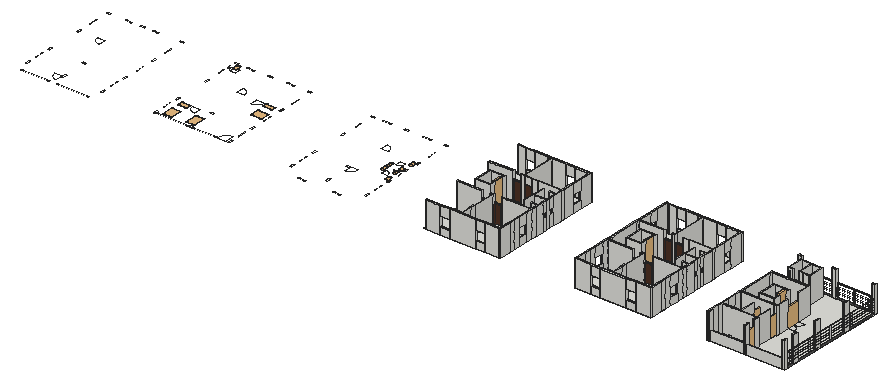
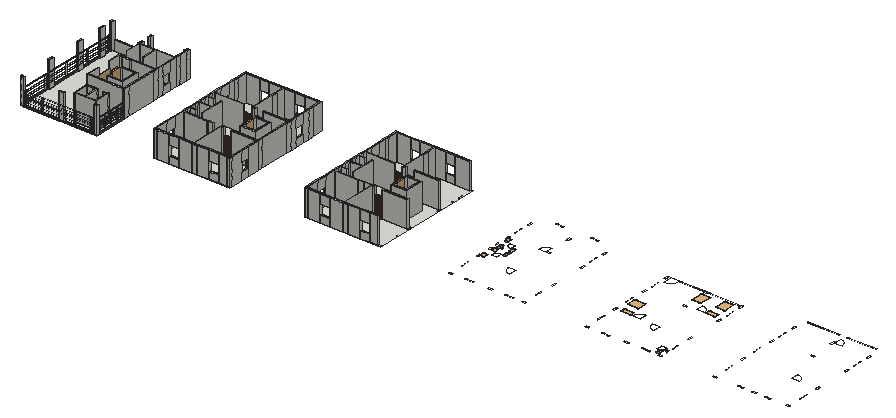
# SketchUp Ruby script. Lengths in inches.
U = 1.inch
M = Sketchup.active_model
def pt(a) = Geom::Point3d.new(a.map { |v| v * U })
def face(e, loops, mat)
  f = e.add_face(loops[0].map { |a| pt(a) })
  loops[1..].each { |l| e.add_face(l.map { |a| pt(a) }).erase! }
  f.material = f.back_material = mat if mat
  f
end
# faces: each face lists its corners as indices into pts; further lists are holes
def faces(e, pts, list, mat = nil) = list.each { |f| face(e, (f[0].is_a?(Array) ? f : [f]).map { |l| l.map { |i| pts[i] } }, mat) }
# xy, xz, yz: faces in a plane at the given z, y or x. An outline is a flat list of corners, or four numbers for a rectangle; further outlines are holes
def ring(l) = l.size == 4 ? [[l[0], l[1]], [l[2], l[1]], [l[2], l[3]], [l[0], l[3]]] : l.each_slice(2).to_a
def flat(e, list, mat, &to3) = list.each { |f| face(e, (f[0].is_a?(Array) ? f : [f]).map { |l| ring(l).map { |u, v| to3.(u, v) } }, mat) }
def xy(e, z, list, mat = nil) = flat(e, list, mat) { |x, y| [x, y, z] }
def xz(e, y, list, mat = nil) = flat(e, list, mat) { |x, z| [x, y, z] }
def yz(e, x, list, mat = nil) = flat(e, list, mat) { |y, z| [x, y, z] }
def lines(e, pts, list) = list.each { |a, b| e.add_line(pt(pts[a]), pt(pts[b])) }
# prism: a flat outline (further loops are holes) pulled along v
def prism(e, loops, v, mat = nil)
  f = face(e, loops, mat); d = Geom::Vector3d.new(v.map { |x| x * U })
  f.pushpull(f.normal.samedirection?(d) ? d.length : -d.length)
end
def box(e, o, s, mat = nil) = prism(e, [[o, [o[0] + s[0], o[1], o[2]], [o[0] + s[0], o[1] + s[1], o[2]], [o[0], o[1] + s[1], o[2]]]], [0, 0, s[2]], mat)
def at(x, y, z, deg = 0) = Geom::Transformation.translation(pt([x, y, z])) * Geom::Transformation.rotation(ORIGIN, Z_AXIS, deg.degrees)
def axes(o, x, y, z) = Geom::Transformation.new([*x, 0, *y, 0, *z, 0, *pt(o).to_a, 1])
def part(name) = M.definitions.add(name)
# library, detail: a bought-in or finely detailed component or shape, given as its bounding box
def library(name, o, s) = part(name).tap { |d| box(d.entities, o, s) }
def detail(e, o, s) = box(e.add_group.entities, o, s)
def put(e, d, t, mat = nil) = e.add_instance(d, t).tap { |i| i.material = mat if mat }
def group(e, t, mat = nil) = e.add_group.tap { |g| g.transformation = t; g.material = mat if mat }.entities
root = M.entities
M.materials.add("JJJ1").color = [238, 218, 183]
M.materials.add("MU TIGHI 6T67L 1").color = [235, 235, 235]
M.materials.add("Polis06_194").color = [79, 50, 36]
M.materials.add("T ER5Y 565N 1").color = [201, 111, 22]
M.materials.add("T R72 56 8, 7 5U1").color = [25, 25, 25]
M.materials.add("wefsd tger 1").color = [92, 92, 92]
c1 = part("bbd")
p = [[-18,-16,0],[-19,-16,0],[18,-16,0],[19,-16,0],[17.2,19.5,0],[14.88,19.37,0],
  [12.57,19.09,0],[10.29,18.67,0],[8.04,18.1,0],[5.83,17.39,0],[3.67,16.53,0],[1.57,15.54,0],
  [-0.46,14.41,0],[-2.41,13.16,0],[-4.28,11.78,0],[-6.0625,10.28,0],[-7.74,8.68,0],[-9.31,6.96,0],
  [-10.76,5.15,0],[-12.1,3.25,0],[-13.31,1.27,0],[-14.39,-0.78,0],[-15.34,-2.9,0],[-16.14,-5.08,0],
  [-16.81,-7.31,0],[-17.33,-9.57,0],[-17.7,-11.86,0],[-17.93,-14.17,0],[-18,-16.5,0],[19.5,-19.5,0],
  [-19.5,-19.5,0],[17,-16.5,0],[18,-16.5,0],[18,19.5,0],[17.2,-16.5,0],[18,-15.5,0],
  [19.5,-15.5,0],[-17,-19.5,0],[-19.5,-15.5,0],[-18,-15.5,0],[-17,-16.5,0],[17,-19.5,0]]
lines(c1.entities,p,[[0,1],[2,3],[4,5],[5,6],[6,7],[7,8],[8,9],[9,10],[10,11],[11,12],[12,13],[13,14],
  [14,15],[15,16],[16,17],[17,18],[18,19],[19,20],[20,21],[21,22],[22,23],[23,24],[24,25],[25,26],
  [26,27],[27,28],[29,30],[31,32],[32,33],[33,4],[4,34],[34,32],[32,35],[35,36],[36,29],[37,30],
  [30,38],[38,39],[39,28],[28,40],[40,37],[31,41],[41,29]])
c2 = part("A$C2CFD65BC")
put(c2.entities,c1,axes([0,0,0],[0.84615,0,0],[0,-0.84615,0],[0,0,0.84615]))
c3 = part("c-1")
p = [[-1.74,-236.76,0],[-12.18,-236.76,0],[-12.18,-260.76,0],[-1.74,-260.76,0],[-184.62,-236.76,0],[-193.62,-236.76,0],
  [-193.62,-260.76,0],[-184.62,-260.76,0],[193.62,-236.76,0],[184.62,-236.76,0],[184.62,-260.76,0],[193.62,-260.76,0],
  [-1.74,-112.8,0],[-1.74,-121.8,0],[-19.74,-121.8,0],[-19.74,-112.8,0],[-175.62,260.76,0],[-175.62,251.76,0],
  [-193.62,251.76,0],[-193.62,260.76,0],[193.62,260.76,0],[193.62,251.76,0],[175.62,251.76,0],[175.62,260.76,0],
  [-1.74,251.76,0],[-1.74,260.76,0],[-25.74,260.76,0],[-25.74,251.76,0],[193.62,-97.8,0],[184.62,-97.8,0],
  [184.62,-121.8,0],[193.62,-121.8,0],[193.62,85.32,0],[184.62,85.32,0],[184.62,61.32,0],[193.62,61.32,0],
  [-184.62,-97.8,0],[-193.62,-97.8,0],[-193.62,-121.8,0],[-184.62,-121.8,0],[-184.62,85.32,0],[-193.62,85.32,0],
  [-193.62,61.32,0],[-184.62,61.32,0]]
lines(c3.entities,p,[[0,1],[1,2],[2,3],[3,0],[4,5],[5,6],[6,7],[7,4],[8,9],[9,10],[10,11],[11,8],
  [12,13],[13,14],[14,15],[15,12],[16,17],[17,18],[18,19],[19,16],[20,21],[21,22],[22,23],[23,20],
  [24,25],[25,26],[26,27],[27,24],[28,29],[29,30],[30,31],[31,28],[32,33],[33,34],[34,35],[35,32],
  [36,37],[37,38],[38,39],[39,36],[40,41],[41,42],[42,43],[43,40]])
c4 = library("A$C064B13D6",[-12.22,-9.4375,0],[24.44,18.875,0.01])
c5 = library("H.F",[-2.42,-4.375,0],[4.84,8.75,0.01])
c6 = library("A$C1C760F31",[-13.95,-18.0625,0],[27.9,36.125,0.01])
c7 = library("A$C4F5E0649",[-23.12,-29.25,0],[46.24,58.5,0.01])
c8 = library("A$C6B07298C",[-24,-12,0],[48,24,0.01])
c9 = library("21''",[-10.5,-8.8125,0],[21,17.625,0.01])
c10 = library("A$C2E2B2BF3",[-14.23,-10.47,0],[28.46,20.94,0.01])
c11 = part("school origo.dwg")
xy(c11.entities,0,[[237.03,315.74,383.625,316.24],[421.44,315.74,584.6,316.24],[1637.66,315.74,1679.3,316.24],[1816.34,315.74,1857.74,316.24],[2364.5625,315.74,2406.2,316.24],
  [2543.24,315.74,2584.64,316.24],[3127,315.74,3168.64,316.24],[3305.68,315.74,3347.08,316.24],[875.22,374.78,1041.66,375.28],[1058.1,374.78,1181.46,375.28],
  [222.16,433.17,222.66,474.57],[600.4,433.17,600.9,474.57],[867.47,433.17,867.97,474.57],[1245.71,433.17,1246.21,474.57],[1556.71,433.17,1557.21,474.57],
  [1934.95,433.17,1935.45,474.57],[2283.61,433.17,2284.11,474.57],[2661.85,433.17,2662.35,474.57],[3046.05,433.17,3046.55,474.57],[3424.29,433.17,3424.79,474.57],
  [3718.02,433.17,3718.52,474.57],[1934.95,581.58,1935.45,599.54],[2661.85,581.58,2662.35,599.54],[3424.29,581.58,3424.79,599.54],[600.4,595.41,600.9,636.81],
  [1245.71,595.41,1246.21,636.81],[1934.95,624.18,1935.45,642.14],[2661.85,624.18,2662.35,642.14],[3424.29,624.18,3424.79,642.14],[222.16,773.125,222.66,814.29],
  [600.4,773.125,600.9,814.29],[1245.71,773.125,1246.21,814.29],[1934.95,773.125,1935.45,814.29],[2661.85,773.125,2662.35,814.29],[3424.29,773.125,3424.79,814.29],
  [867.47,784.33,867.97,814.29],[1556.71,784.33,1557.21,814.29],[2283.61,784.33,2284.11,814.29],[3046.05,784.33,3046.55,814.29],[867.47,835.87,867.97,853.83],
  [315.11,887.3,344.75,887.8],[450.83,887.3,480.23,887.8],[925.02,887.3,966.66,887.8],[1127.1,887.3,1168.5,887.8],[1614.26,887.3,1655.9,887.8],
  [1816.34,887.3,1857.74,887.8],[2341.16,887.3,2382.8,887.8],[2543.24,887.3,2584.64,887.8],[3103.6,887.3,3145.24,887.8],[3305.68,887.3,3347.08,887.8]])
# 6092 loose lines left out
put(c11.entities,c2,axes([3883.4375,490.05,0],[0,1.17818,0],[1.17818,0,0],[0,0,1.17818]))
put(c11.entities,c2,axes([2433.74,727.1,0],[1.18182,0,0],[0,-1.18182,0],[0,0,1.18182]))
put(c11.entities,c2,axes([1763.84,498.99,0],[-1.18182,0,0],[0,1.18182,0],[0,0,1.18182]))
put(c11.entities,c3,at(1746.08,631.29,0))
put(c11.entities,c3,at(3908.89,631.29,0))
put(c11.entities,c3,at(1056.84,631.29,0))
put(c11.entities,c3,at(411.53,631.29,0))
put(c11.entities,c2,axes([333.42,688.11,0],[0,1.18182,0],[1.18182,0,0],[0,0,1.18182]))
put(c11.entities,c2,axes([379.85,360.03,0],[1.18182,0,0],[0,1.18182,0],[0,0,1.18182]))
put(c11.entities,c2,axes([902.52,838.82,0],[0.90909,0,0],[0,-0.90909,0],[0,0,0.90909]))
put(c11.entities,c4,at(894.87,862.82,0,90))
put(c11.entities,c5,axes([875.21,841.2,0],[0,-0.68414,0],[-0.68414,0,0],[0,0,0.68414]))
put(c11.entities,c2,axes([1035.6,727.1,0],[-1.18182,0,0],[0,-1.18182,0],[0,0,1.18182]))
put(c11.entities,c2,axes([1208.46,394.52,0],[1.45455,0,0],[0,-1.45455,0],[0,0,1.45455]))
put(c11.entities,c6,axes([1031.8,427.7,0],[-1.6702,0,0],[0,-1.6702,0],[0,0,1.6702]))
put(c11.entities,c2,axes([972.81,490.07,0],[0,1.17684,0],[1.17684,0,0],[0,0,1.17684]))
put(c11.entities,c7,at(920.83,419.28,0))
put(c11.entities,c8,at(921.75,496.49,0))
put(c11.entities,c2,axes([1763.84,727.1,0],[-1.18182,0,0],[0,-1.18182,0],[0,0,1.18182]))
put(c11.entities,c9,axes([1912.68,631.8,0],[0,1,0],[1,0,0],[0,0,1]))
put(c11.entities,c5,axes([1927.7,624.29,0],[0.68414,0,0],[0,-0.68414,0],[0,0,0.68414]))
put(c11.entities,c10,axes([1921.87,536.4375,0],[0,0.84313,0],[0.84313,0,0],[0,0,0.84313]))
put(c11.entities,c9,axes([1912.72,594.3,0],[0,-1,0],[-1,0,0],[0,0,1]))
put(c11.entities,c5,axes([1897.7,601.8,0],[-0.68414,0,0],[0,0.68414,0],[0,0,0.68414]))
put(c11.entities,c2,axes([1885.7,569.48,0],[-0.90909,0,0],[0,-0.90909,0],[0,0,0.90909]))
put(c11.entities,c2,axes([3920.65,631.05,0],[0,1.09091,0],[-1.09091,0,0],[0,0,1.09091]))
put(c11.entities,c2,axes([3920.65,595.05,0],[0,-1.09091,0],[-1.09091,0,0],[0,0,1.09091]))
put(c11.entities,c2,axes([1137.96,688.11,0],[0,1.18182,0],[-1.18182,0,0],[0,0,1.18182]))
put(c11.entities,c7,at(1201.71,623.01,0,90))
put(c11.entities,c8,axes([1191.82,693.61,0],[-1,0,0],[0,1,0],[0,0,1]))
put(c11.entities,c2,axes([1885.7,656.61,0],[-0.90909,0,0],[0,0.90909,0],[0,0,0.90909]))
put(c11.entities,c10,axes([1921.87,689.56,0],[0,0.84313,0],[0.84313,0,0],[0,0,0.84313]))
put(c11.entities,c10,axes([1854.72,593.92,0],[0,0.84313,0],[0.84313,0,0],[0,0,0.84313]))
put(c11.entities,c10,axes([1854.72,632.17,0],[0,-0.84313,0],[0.84313,0,0],[0,0,0.84313]))
put(c11.entities,c2,axes([2490.74,498.99,0],[-1.18182,0,0],[0,1.18182,0],[0,0,1.18182]))
put(c11.entities,c3,at(2472.98,631.29,0))
put(c11.entities,c2,axes([2490.74,727.1,0],[-1.18182,0,0],[0,-1.18182,0],[0,0,1.18182]))
put(c11.entities,c9,axes([2639.58,631.8,0],[0,1,0],[1,0,0],[0,0,1]))
put(c11.entities,c5,axes([2654.6,624.29,0],[0.68414,0,0],[0,-0.68414,0],[0,0,0.68414]))
put(c11.entities,c10,axes([2648.77,536.4375,0],[0,0.84313,0],[0.84313,0,0],[0,0,0.84313]))
put(c11.entities,c9,axes([2639.625,594.3,0],[0,-1,0],[-1,0,0],[0,0,1]))
put(c11.entities,c5,axes([2624.6,601.8,0],[-0.68414,0,0],[0,0.68414,0],[0,0,0.68414]))
put(c11.entities,c2,axes([2612.6,569.48,0],[-0.90909,0,0],[0,-0.90909,0],[0,0,0.90909]))
put(c11.entities,c2,axes([2612.6,656.61,0],[-0.90909,0,0],[0,0.90909,0],[0,0,0.90909]))
put(c11.entities,c10,axes([2648.77,689.56,0],[0,0.84313,0],[0.84313,0,0],[0,0,0.84313]))
put(c11.entities,c10,axes([2581.62,593.92,0],[0,0.84313,0],[0.84313,0,0],[0,0,0.84313]))
put(c11.entities,c10,axes([2581.62,632.17,0],[0,-0.84313,0],[0.84313,0,0],[0,0,0.84313]))
put(c11.entities,c2,axes([2433.74,498.99,0],[1.18182,0,0],[0,1.18182,0],[0,0,1.18182]))
put(c11.entities,c2,axes([3196.18,727.1,0],[1.18182,0,0],[0,-1.18182,0],[0,0,1.18182]))
put(c11.entities,c2,axes([3253.18,498.99,0],[-1.18182,0,0],[0,1.18182,0],[0,0,1.18182]))
put(c11.entities,c3,at(3235.42,631.29,0))
put(c11.entities,c2,axes([3253.18,727.1,0],[-1.18182,0,0],[0,-1.18182,0],[0,0,1.18182]))
put(c11.entities,c9,axes([3402.01,631.8,0],[0,1,0],[1,0,0],[0,0,1]))
put(c11.entities,c5,axes([3417.04,624.29,0],[0.68414,0,0],[0,-0.68414,0],[0,0,0.68414]))
put(c11.entities,c10,axes([3411.2,536.4375,0],[0,0.84313,0],[0.84313,0,0],[0,0,0.84313]))
put(c11.entities,c9,axes([3402.06,594.3,0],[0,-1,0],[-1,0,0],[0,0,1]))
put(c11.entities,c5,axes([3387.04,601.8,0],[-0.68414,0,0],[0,0.68414,0],[0,0,0.68414]))
put(c11.entities,c2,axes([3375.04,569.48,0],[-0.90909,0,0],[0,-0.90909,0],[0,0,0.90909]))
put(c11.entities,c2,axes([3375.04,656.61,0],[-0.90909,0,0],[0,0.90909,0],[0,0,0.90909]))
put(c11.entities,c10,axes([3411.2,689.56,0],[0,0.84313,0],[0.84313,0,0],[0,0,0.84313]))
put(c11.entities,c10,axes([3344.05,593.92,0],[0,0.84313,0],[0.84313,0,0],[0,0,0.84313]))
put(c11.entities,c10,axes([3344.05,632.17,0],[0,-0.84313,0],[0.84313,0,0],[0,0,0.84313]))
put(c11.entities,c2,axes([3196.18,498.99,0],[1.18182,0,0],[0,1.18182,0],[0,0,1.18182]))
put(c11.entities,c2,axes([3884.88,352.53,0],[0,1.09091,0],[1.09091,0,0],[0,0,1.09091]))
put(c11.entities,c2,axes([3783.02,797.04,0],[0.90909,0,0],[0,-0.90909,0],[0,0,0.90909]))
put(c11.entities,c2,axes([3836.02,797.04,0],[0.90909,0,0],[0,-0.90909,0],[0,0,0.90909]))
put(c11.entities,c4,at(3774.52,837.82,0,90))
put(c11.entities,c5,axes([3754.02,816.2,0],[0,-0.68414,0],[-0.68414,0,0],[0,0,0.68414]))
put(c11.entities,c4,at(3827.52,837.82,0,90))
put(c11.entities,c5,axes([3807.02,816.2,0],[0,-0.68414,0],[-0.68414,0,0],[0,0,0.68414]))
put(c11.entities,c2,axes([3801.14,490.05,0],[0,1.17818,0],[1.17818,0,0],[0,0,1.17818]))
c12 = library("lift",[-933.37,365.14,432],[57.92,12.32,108.27])
c13 = part("Group\#210")
box(c13.entities,[0,0,0],[12,46.92,6])
c14 = part("Flush door assembly \#1")
xy(c14.entities,0,[[0,0,4.72,1.18],[0,34.25,4.72,35.43]],"Polis06_194")
xy(c14.entities,85.26,[[0,1.18,4.72,34.25]],"Polis06_194")
xy(c14.entities,86.61,[[0,0,4.72,35.43]],"Polis06_194")
xz(c14.entities,0,[[0,0,4.72,86.61]],"Polis06_194")
xz(c14.entities,1.18,[[0,0,2.36,85.26],[2.36,0,4.72,85.26]],"Polis06_194")
xz(c14.entities,34.25,[[0,0,4.72,85.26]],"Polis06_194")
xz(c14.entities,35.43,[[0,0,4.72,86.61]],"Polis06_194")
yz(c14.entities,0,[[0,0,1.18,86.61],[34.25,0,35.43,86.61],[1.18,85.26,34.25,86.61]],"Polis06_194")
yz(c14.entities,2.36,[[1.18,0,34.25,0,34.25,85.21,1.18,85.26]],"Polis06_194")
yz(c14.entities,4.72,[[0,0,1.18,86.61],[34.25,0,35.43,86.61],[1.18,85.26,34.25,86.61]],"Polis06_194")
c15 = library("Flush door assembly",[0,0,0],[5.12,30.08,83.9375])
c16 = part("Group\#154")
box(c16.entities,[0,0,0],[12,46.92,6])
c17 = part("Box01")
box(c17.entities,[-251.12,-5.93,-8.91],[582.61,12.27,8.91],"wefsd tger 1")
c18 = part("Box45")
box(c18.entities,[-240.91,-0.82,12.1],[2.44,1.82,74.48],"JJJ1")
c19 = part("Cylinder01")
prism(c19.entities,[[[328.21,-1.16,98.56],[328.21,-0.34,98.26],[328.21,0.53,98.26],[328.21,1.34,98.56],[328.21,2.01,99.11],[328.21,2.44,99.87],[328.21,2.59,100.72],[328.21,2.44,101.58],[328.21,2.01,102.33],[328.21,1.34,102.89],[328.21,0.53,103.18],[328.21,-0.34,103.18],[328.21,-1.16,102.89],[328.21,-1.82,102.33],[328.21,-2.25,101.58],[328.21,-2.41,100.72],[328.21,-2.25,99.87],[328.21,-1.82,99.11]]],[-576.3,0,0],"T ER5Y 565N 1")
c20 = part("Cylinder02")
prism(c20.entities,[[[-239.93,0.18,76.32],[-239.93,0.34,76.26],[-239.93,0.48,76.15],[-239.93,0.5625,75.99],[-239.93,0.59,75.82],[-239.93,0.5625,75.65],[-239.93,0.48,75.5],[-239.93,0.34,75.39],[-239.93,0.18,75.33],[-239.93,0.01,75.33],[-239.93,-0.16,75.39],[-239.93,-0.29,75.5],[-239.93,-0.375,75.65],[-239.93,-0.41,75.82],[-239.93,-0.375,75.99],[-239.93,-0.29,76.15],[-239.93,-0.16,76.26],[-239.93,0.01,76.32]]],[560.05,0,0],"T R72 56 8, 7 5U1")
c21 = part("Rectangle1")
prism(c21.entities,[[[-237.41,1.91,10.08],[-239.22,1.91,10.08],[-239.22,1.91,0.02],[-240.41,1.91,0.02],[-240.41,1.91,10.08],[-242.22,1.91,10.08],[-242.22,1.91,89.41],[-240.41,1.91,89.41],[-240.41,1.91,99.1875],[-239.22,1.91,99.1875],[-239.22,1.91,89.41],[-237.41,1.91,89.41]],[[-240.4375,1.91,85.68],[-240.4375,1.91,13.53],[-239.08,1.91,13.53],[-239.08,1.91,85.68]]],[0,-3.64,0],"MU TIGHI 6T67L 1")
c22 = part("skp243")
put(c22.entities,c17,at(0,0,0))
put(c22.entities,c18,at(0,0,0))
put(c22.entities,c19,at(0,0,0))
put(c22.entities,c20,at(0,0,0))
put(c22.entities,c21,at(0,0,0))
put(c22.entities,c20,at(0,0,-17.07))
put(c22.entities,c20,at(0,0,-35.38))
put(c22.entities,c20,at(0,0,-53.15))
put(c22.entities,c18,at(139.83,0,0))
put(c22.entities,c21,at(139.83,0,0))
put(c22.entities,c21,at(279.78,0,0))
put(c22.entities,c18,at(279.78,0,0))
put(c22.entities,c18,at(419.57,0,0))
put(c22.entities,c21,at(419.57,0,0))
put(c22.entities,c21,at(561.11,0,0))
put(c22.entities,c18,at(561.11,0,0))
c23 = part("Railing1 (1)")
put(c23.entities,c22,at(251.12,5.93,8.91))
c24 = part("Group\#105")
box(c24.entities,[0,0,0],[12,46.92,6])
c25 = library("DD LT 2",[0,0,0],[47.24,4.7,78.74])
xy(root,0,[[2061.45,72,2448.69,652.56],[2823.88,72,3211.125,652.56],[3497.36,72,3884.6,652.56]])
g1 = group(root,at(2079.45,643.56,0))
box(g1,[0,0,0],[40.8,9,132])
put(root,c11,at(-217.91,-239.49,0))
g2 = group(root,at(2070.45,72,0))
box(g2,[0,0,0],[73.2,9,132])
g3 = group(root,at(2070.45,468.12,0))
box(g3,[0,0,0],[125.88,9,132])
g4 = group(root,at(2070.45,270,0))
box(g4,[0,0,0],[126,9,132])
g5 = group(root,at(2120.25,643.56,0))
box(g5,[0,0,0],[47.64,9,36])
box(g5,[0,0,84],[47.64,9,48])
# 2 loose lines left out
g6 = group(root,at(2117.37,325.92,0))
prism(g6,[[[9,9,0],[70.08,9,0],[70.08,29.64,0],[79.08,29.64,0],[79.08,0,0],[0,0,0],[0,95.28,0],[79.08,95.28,0],[79.08,65.64,0],[70.08,65.64,0],[70.08,86.28,0],[9,86.28,0]]],[0,0,132])
g7 = group(root,at(2143.65,72,0))
box(g7,[0,0,0],[47.64,9,36])
box(g7,[0,0,84],[47.64,9,48])
# 2 loose lines left out
put(root,c12,axes([2561.59,1008.92,-527.04],[0,0.7,0],[-1,0,0],[0,0,1.22]))
put(root,c13,at(2184.45,279,0))
g8 = group(root,at(2167.89,643.56,0))
box(g8,[0,0,0],[61.44,9,132])
put(root,c14,axes([2235.33,468.12,0],[0,1,0],[-1.10067,0,0],[0,0,1.10836]))
put(root,c14,axes([2235.33,270,0],[0,1,0],[-1.10067,0,0],[0,0,1.10836]))
g9 = group(root,at(2229.33,643.56,0))
box(g9,[0,0,0],[24,9,132])
g10 = group(root,at(2235.33,468.12,0))
prism(g10,[[[0,0,0],[0,9,0],[14,9,0],[18,9,0],[18,0,0]]],[0,0,132])
g11 = group(root,at(2235.33,270,0))
box(g11,[0,0,0],[18,9,132])
g12 = group(root,at(2242.89,131.04,0))
box(g12,[0,0,0],[10.44,24,132])
g13 = group(root,at(2249.33,477.12,0))
box(g13,[0,0,0],[4,166.44,132])
g14 = group(root,at(2249.33,81,0))
box(g14,[0,0,0],[4,50.04,132])
g15 = group(root,at(2249.33,155.04,0))
box(g15,[0,0,0],[4,114.96,132])
g16 = group(root,at(2191.29,72,0))
prism(g16,[[[62.04,9,0],[131.04,9,0],[131.04,0,0],[0,0,0],[0,9,0],[58.04,9,0]]],[0,0,132])
put(root,c14,axes([2292.33,468.12,0],[0,1,0],[-1.10067,0,0],[0,0,1.10836]))
put(root,c14,axes([2292.33,275,0],[0,1,0],[-1.10067,0,0],[0,0,1.10836]))
g17 = group(root,at(2253.33,468.12,0))
box(g17,[0,0,96],[39,3,36])
# 3 loose lines left out
g18 = group(root,at(2253.33,643.56,0))
box(g18,[0,0,0],[69,9,132])
g19 = group(root,at(2292.33,468.12,0))
box(g19,[0,0,0],[29.36,3,132])
g20 = group(root,at(2322.33,72,0))
box(g20,[0,0,0],[47.4,9,36])
box(g20,[0,0,84],[47.4,9,48])
# 2 loose lines left out
g21 = group(root,at(2322.33,643.56,0))
box(g21,[0,0,0],[47.4,9,36])
box(g21,[0,0,84],[47.4,9,48])
# 2 loose lines left out
g22 = group(root,at(2292.33,275,0))
box(g22,[0,0,0],[147.36,4,132])
g23 = group(root,at(2375.19,315,0))
prism(g23,[[[4.5,117.12,0],[4.5,60.81,0],[4.5,56.31,0],[4.5,0,0],[0,0,0],[0,117.12,0]]],[0,0,132])
g24 = group(root,at(2321.69,468.12,0))
prism(g24,[[[0,4.5,0],[118,4.5,0],[118,0,0],[0,0,0],[0,3,0]]],[0,0,132])
put(root,c15,at(2409.69,315,0,90))
put(root,c15,at(2409.69,427.62,0,90))
g25 = group(root,at(2369.73,643.56,0))
box(g25,[0,0,0],[60.96,9,132])
g26 = group(root,at(2369.73,72,0))
box(g26,[0,0,0],[69.96,9,132])
g27 = group(root,at(2379.69,371.31,0))
box(g27,[0,0,0],[60,4.5,132])
g28 = group(root,at(2409.69,315,0))
box(g28,[0,0,0],[30,4.5,132])
g29 = group(root,at(2409.69,427.62,0))
box(g29,[0,0,0],[30,4.5,132])
g30 = group(root,at(2430.69,643.56,0))
box(g30,[0,0,0],[18,9,132])
g31 = group(root,at(2439.69,381.66,0))
box(g31,[0,0,0],[9,24,60])
box(g31,[0,0,84],[9,24,48])
# 2 loose lines left out
g32 = group(root,at(2439.69,72,0))
prism(g32,[[[9,0,0],[0,0,0],[0,9,0],[0,59.04,0],[9,59.04,0]]],[0,0,132])
g33 = group(root,at(2439.69,294,0))
prism(g33,[[[0,45.05,0],[9,45.05,0],[9,0,0],[0,0,0],[0,21,0],[0,25.5,0]]],[0,0,132])
g34 = group(root,at(2439.69,363.05,0))
prism(g34,[[[9,0,0],[0,0,0],[0,8.26,0],[0,12.76,0],[0,18.61,0],[9,18.61,0]]],[0,0,132])
g35 = group(root,at(2439.69,339.05,0))
box(g35,[0,0,0],[9,24,60])
box(g35,[0,0,84],[9,24,48])
g36 = group(root,at(2439.69,155.04,0))
box(g36,[0,0,0],[9,35.64,132])
g37 = group(root,at(2439.69,238.08,0))
box(g37,[0,0,0],[9,31.92,132])
g38 = group(root,at(2439.69,405.66,0))
prism(g38,[[[0,0,0],[0,21.96,0],[0,26.46,0],[0,47.46,0],[9,47.46,0],[9,0,0]]],[0,0,132])
g39 = group(root,at(2439.69,477.12,0))
box(g39,[0,0,0],[9,53.52,132])
g40 = group(root,at(2439.69,530.64,0))
box(g40,[0,0,0],[9,47.16,36])
box(g40,[0,0,84],[9,47.16,48])
# 2 loose lines left out
g41 = group(root,at(2439.69,190.68,0))
box(g41,[0,0,0],[9,47.4,36])
box(g41,[0,0,84],[9,47.4,48])
# 2 loose lines left out
g42 = group(root,at(2439.69,131.04,0))
box(g42,[0,0,0],[9,24,132])
g43 = group(root,at(2439.69,270,0))
box(g43,[0,0,0],[9,24,132])
g44 = group(root,at(2439.69,453.12,0))
box(g44,[0,0,0],[9,24,132])
g45 = group(root,at(2439.69,577.8,0))
box(g45,[0,0,0],[9,65.76,132])
g46 = group(root,at(2823.88,541.88,0))
prism(g46,[[[9,0,0],[9,35.92,0],[9,35.92,36],[9,0.68,36],[9,0.68,84],[9,35.92,84],[9,35.92,132],[9,0,132]]],[-9,0,0])
g47 = group(root,at(2823.88,238.08,0))
box(g47,[0,0,0],[9,31.92,132])
g48 = group(root,at(2823.88,190.68,0))
box(g48,[0,0,0],[9,47.4,36])
box(g48,[0,0,84],[9,47.4,48])
# 2 loose lines left out
g49 = group(root,at(2823.88,477.12,0))
box(g49,[0,0,0],[9,64.76,132])
g50 = group(root,at(2823.88,577.8,0))
box(g50,[0,0,0],[9,65.76,132])
g51 = group(root,at(2823.88,453.12,0))
box(g51,[0,0,0],[9,24,132])
g52 = group(root,at(2823.88,270,0))
box(g52,[0,0,0],[9,24,132])
g53 = group(root,at(2823.88,131.04,0))
box(g53,[0,0,0],[9,24,132])
g54 = group(root,at(2823.88,294,0))
box(g54,[0,0,0],[9,159.12,132])
g55 = group(root,at(2823.88,155.04,0))
box(g55,[0,0,0],[9,35.64,132])
g56 = group(root,at(2823.88,643.56,0))
box(g56,[0,0,0],[18,9,132])
g57 = group(root,at(2841.88,643.56,0))
box(g57,[0,0,0],[40.8,9,132])
g58 = group(root,at(2823.88,72,0))
prism(g58,[[[82.2,0,0],[0,0,0],[0,59.04,0],[9,59.04,0],[9,9,0],[82.2,9,0]]],[0,0,132])
g59 = group(root,at(2832.88,468.12,0))
box(g59,[0,0,0],[125.88,9,132])
g60 = group(root,at(2832.88,270,0))
box(g60,[0,0,0],[126,9,132])
g61 = group(root,at(2882.68,643.56,0))
box(g61,[0,0,0],[47.64,9,36])
box(g61,[0,0,84],[47.64,9,48])
# 2 loose lines left out
g62 = group(root,at(2879.8,325.92,0))
prism(g62,[[[0,95.28,0],[79.08,95.28,0],[79.08,65.64,0],[70.08,65.64,0],[70.08,86.28,0],[9,86.28,0],[9,9,0],[70.08,9,0],[70.08,29.64,0],[79.08,29.64,0],[79.08,0,0],[0,0,0]]],[0,0,132])
g63 = group(root,at(2906.08,72,0))
xy(g63,0,[[0,0,47.64,9]])
xy(g63,36,[[0,0,47.64,9],[0,9,47.64,9.65]])
xy(g63,84,[[0,0,47.64,9],[0,9,47.64,9.65]])
xy(g63,132,[[0,0,47.64,9]])
xz(g63,0,[[0,0,47.64,36],[0,84,47.64,132]])
xz(g63,9,[[0,0,47.64,36],[0,84,47.64,132]])
yz(g63,0,[[0,0,9,36],[0,84,9,132]])
yz(g63,47.64,[[0,0,9,36],[0,84,9,132]])
put(root,c12,axes([3324.03,1008.92,-527.04],[0,0.7,0],[-1,0,0],[0,0,1.22]))
put(root,c16,at(2946.88,279,0))
g64 = group(root,at(2930.32,643.56,0))
box(g64,[0,0,0],[61.44,9,132])
put(root,c14,axes([2997.76,468.12,0],[0,1,0],[-1.10067,0,0],[0,0,1.10836]))
put(root,c14,axes([2997.76,270,0],[0,1,0],[-1.10067,0,0],[0,0,1.10836]))
g65 = group(root,at(2991.76,643.56,0))
box(g65,[0,0,0],[24,9,132])
g66 = group(root,at(2997.76,270,0))
box(g66,[0,0,0],[18,9,132])
g67 = group(root,at(2997.76,468.12,0))
prism(g67,[[[18,9,0],[18,0,0],[0,0,0],[0,9,0],[14,9,0]]],[0,0,132])
g68 = group(root,at(3005.32,131.04,0))
box(g68,[0,0,0],[10.44,24,132])
g69 = group(root,at(3011.76,81,0))
box(g69,[0,0,0],[4,50.04,132])
g70 = group(root,at(3011.76,477.12,0))
box(g70,[0,0,0],[4,166.44,132])
g71 = group(root,at(3011.76,155.04,0))
box(g71,[0,0,0],[4,114.96,132])
g72 = group(root,at(2953.72,72,0))
prism(g72,[[[0,0,0],[0,9,0],[58.04,9,0],[62.04,9,0],[131.04,9,0],[131.04,0,0]]],[0,0,132])
put(root,c14,axes([3054.76,468.12,0],[0,1,0],[-1.10067,0,0],[0,0,1.10836]))
put(root,c14,axes([3054.76,275,0],[0,1,0],[-1.10067,0,0],[0,0,1.10836]))
g73 = group(root,at(3015.76,643.56,0))
box(g73,[0,0,0],[69,9,132])
g74 = group(root,at(3054.76,468.12,0))
box(g74,[0,0,0],[29.36,3,132])
g75 = group(root,at(3084.76,72,0))
box(g75,[0,0,0],[47.4,9,36])
box(g75,[0,0,84],[47.4,9,48])
# 2 loose lines left out
g76 = group(root,at(3084.76,643.56,0))
box(g76,[0,0,0],[47.4,9,36])
box(g76,[0,0,84],[47.4,9,48])
# 2 loose lines left out
g77 = group(root,at(3054.76,275,0))
box(g77,[0,0,0],[147.36,4,132])
g78 = group(root,at(3137.625,315,0))
prism(g78,[[[4.5,56.31,0],[4.5,0,0],[0,0,0],[0,117.12,0],[4.5,117.12,0],[4.5,60.81,0]]],[0,0,132])
g79 = group(root,at(3084.125,468.12,0))
prism(g79,[[[0,3,-0.64],[0,4.5,-0.64],[118,4.5,-0.64],[118,0,-0.64],[0,0,-0.64]]],[0,0,132.64])
put(root,c15,at(3172.125,430.45,0,90))
put(root,c15,at(3172.125,315,0,90))
g80 = group(root,at(3132.16,643.56,0))
box(g80,[0,0,0],[60.96,9,132])
g81 = group(root,at(3132.16,72,0))
prism(g81,[[[78.96,0,0],[0,0,0],[0,9,0],[69.96,9,0],[78.96,9,0]]],[0,0,132])
g82 = group(root,at(3142.125,371.31,0))
box(g82,[0,0,0],[60,4.5,132])
g83 = group(root,at(3172.125,427.62,0))
box(g83,[0,0,0],[30,4.5,132])
g84 = group(root,at(3172.125,315,0))
box(g84,[0,0,0],[30,4.5,132])
g85 = group(root,at(3193.125,643.56,0))
box(g85,[0,0,0],[18,9,132])
g86 = group(root,at(3202.125,577.8,0))
box(g86,[0,0,0],[9,65.76,132])
g87 = group(root,at(3202.125,530.64,0))
box(g87,[0,0,0],[9,47.16,36])
box(g87,[0,0,84],[9,47.16,48])
# 2 loose lines left out
g88 = group(root,at(3202.125,190.68,0))
box(g88,[0,0,0],[9,47.4,36])
box(g88,[0,0,84],[9,47.4,48])
# 2 loose lines left out
g89 = group(root,at(3202.125,155.04,0))
box(g89,[0,0,0],[9,35.64,132])
g90 = group(root,at(3202.125,238.08,0))
box(g90,[0,0,0],[9,31.92,132])
g91 = group(root,at(3202.125,477.12,0))
box(g91,[0,0,0],[9,53.52,132])
g92 = group(root,at(3202.125,405.66,0))
prism(g92,[[[9,0,0],[0,0,0],[0,21.96,0],[0,26.46,0],[0,47.46,0],[9,47.46,0]]],[0,0,132])
g93 = group(root,at(3202.125,81,0))
box(g93,[0,0,0],[9,50.04,132])
g94 = group(root,at(3202.125,453.12,0))
box(g94,[0,0,0],[9,24,132])
g95 = group(root,at(3202.125,270,0))
box(g95,[0,0,0],[9,24,132])
g96 = group(root,at(3202.125,131.04,0))
box(g96,[0,0,0],[9,24,132])
g97 = group(root,at(3202.125,363.05,0))
prism(g97,[[[9,18.65,0],[9,0,0],[0,0,0],[0,8.26,0],[0,12.76,0],[0,18.65,0]]],[0,0,132])
g98 = group(root,at(3202.125,381.7,0))
box(g98,[0,0,0],[9,23.96,60])
box(g98,[0,0,84],[9,23.96,48])
# 2 loose lines left out
g99 = group(root,at(3202.125,294,0))
prism(g99,[[[9,45.09,0],[9,0,0],[0,0,0],[0,21,0],[0,25.5,0],[0,45.09,0]]],[0,0,132])
g100 = group(root,at(3202.125,339.09,0))
box(g100,[0,0,0],[9,23.96,60])
box(g100,[0,0,84],[9,23.96,48])
# 2 loose lines left out
put(root,c23,axes([3502.52,477.12,0],[0,0.28568,0],[-0.42,0,0],[0,0,0.648]))
g101 = group(root,at(3497.36,238.08,0))
box(g101,[0,0,0],[6,31.92,132])
g102 = group(root,at(3497.36,190.68,0))
box(g102,[0,0,0],[6,47.4,36])
box(g102,[0,0,84],[6,47.4,48])
# 2 loose lines left out
g103 = group(root,at(3497.36,477.12,0))
xy(g103,0,[[0,0,6,166.44]])
g104 = group(root,at(3497.36,155.04,0))
box(g104,[0,0,0],[6,35.64,132])
g105 = group(root,at(3497.36,85.32,0))
box(g105,[0,0,0],[6,45.72,132])
g106 = group(root,at(3497.36,131.04,0))
box(g106,[0,0,0],[9,24,132])
g107 = group(root,at(3497.36,270,0))
box(g107,[0,0,0],[9,24,131.82])
g108 = group(root,at(3497.36,453.12,0))
box(g108,[0,0,0],[9,24,132])
g109 = group(root,at(3497.36,294,0))
box(g109,[0,0,0],[9,159.12,132])
g110 = group(root,at(3497.36,67,0))
prism(g110,[[[9,0,0],[0,0,0],[0,18.32,0],[12.6,18.32,0],[12.6,5,0],[9.3,5,0],[9,5,0]]],[0,0,132])
g111 = group(root,at(3497.36,643.56,0))
box(g111,[0,0,0],[18,9,132])
g112 = group(root,at(3527.11,548.56,0))
box(g112,[0,0,0],[6,70,132])
g113 = group(root,at(3527.11,542.56,0))
prism(g113,[[[6,6,0],[23,6,0],[23,0,0],[0,0,0],[0,6,0]]],[0,0,132])
put(root,c15,at(3580.11,542.56,0,90))
g114 = group(root,at(3527.11,618.56,0))
prism(g114,[[[0,0,0],[0,6,0],[106,6,0],[106,0,0],[59,0,0],[53,0,0],[6,0,0]]],[0,0,132])
g115 = group(root,at(3580.11,548.56,0))
box(g115,[0,0,0],[6,70,132])
g116 = group(root,at(3506.36,270,0))
prism(g116,[[[126,9,0],[164.88,9,0],[164.88,0,0],[0,0,0],[0,9,0],[120,9,0]]],[0,0,132])
g117 = group(root,at(3515.36,646.56,0))
xy(g117,0,[[0,0,149.88,6]])
g118 = group(root,at(3580.11,542.56,0))
prism(g118,[[[23,6,0],[23,0,0],[0,0,0],[0,6,0],[6,6,0]]],[0,0,132])
g119 = group(root,at(3506.36,150.54,0))
prism(g119,[[[0,0,0],[0,4.5,0],[91.8,4.5,0],[96.3,4.5,0],[172.44,4.5,0],[172.44,0,0]]],[0,0,132])
g120 = group(root,at(3553.28,325.92,0))
prism(g120,[[[79.08,95.28,0],[79.08,65.64,0],[70.08,65.64,0],[70.08,86.28,0],[9,86.28,0],[9,9,0],[70.08,9,0],[70.08,29.64,0],[79.08,29.64,0],[79.08,0,0],[73.08,0,0],[0,0,0],[0,95.28,0]]],[0,0,120])
g121 = group(root,at(3509.96,72,0))
prism(g121,[[[92.5,6,0],[171,6,0],[171,0,0],[0,0,0],[0,6,0],[82.5,6,0],[82.5,13.32,0],[92.5,13.32,0]]],[0,0,48])
g122 = group(root,at(3506.36,409.56,0))
prism(g122,[[[178.38,58.56,0],[0,58.56,0],[0,67.56,0],[182.88,67.56,0],[182.88,0,0],[178.38,0,0]]],[0,0,132])
put(root,c15,axes([3602.66,270,0],[-1,0,0],[0,-1.28286,0],[0,0,1.14371]))
g123 = group(root,at(3598.16,155.04,0))
box(g123,[0,0,0],[4.5,76.08,132])
put(root,c15,at(3633.11,542.56,0,90))
g124 = group(root,at(3603.11,542.56,0))
box(g124,[0,0,84],[30,6,48])
# 3 loose lines left out
put(root,c12,axes([3997.5,1008.92,-527.04],[0,0.7,0],[-1,0,0],[0,0,1.22]))
put(root,c24,at(3620.36,279,0))
g125 = group(root,at(3633.11,542.56,0))
prism(g125,[[[0,82,0],[6,82,0],[6,0,0],[0,0,0],[0,76,0]]],[0,0,132])
g126 = group(root,at(3665.24,643.56,0))
box(g126,[0,0,0],[24,9,132])
g127 = group(root,at(3671.24,270,0))
box(g127,[0,0,0],[18,9,131.82])
put(root,c15,axes([3683.92,131.04,0],[-1,0,0],[0,-1.2,0],[0,0,1.14371]))
put(root,c15,axes([3683.92,270,0],[-1,0,0],[0,-1.28286,0],[0,0,1.14371]))
g128 = group(root,at(3680.96,155.04,0))
box(g128,[0,0,0],[4,76.08,132])
g129 = group(root,at(3680.96,87,0))
box(g129,[0,0,0],[4,8.04,132])
g130 = group(root,at(3678.8,131.04,0))
box(g130,[0,0,0],[10.44,24,132])
g131 = group(root,at(3680.96,72,0))
box(g131,[0,0,0],[10,15,131.82])
put(root,c25,axes([3689.24,337.56,0],[0,1.524,0],[-1,0,0],[0,0,1.224]))
g132 = group(root,at(3684.74,279,0))
box(g132,[0,0,0],[4.5,58.56,132])
put(root,c23,axes([3515.36,647.41,0],[0.60287,0,0],[0,0.42,0],[0,0,0.648]))
g133 = group(root,at(3768.46,78,0))
xy(g133,0,[[0,0,10,4.5]])
g134 = group(root,at(3689.24,646.56,0))
xy(g134,0,[[0,0,177.36,6]])
g135 = group(root,at(3690.96,72,0))
box(g135,[0,0,0],[182.64,6,48])
g136 = group(root,at(3866.6,643.56,0))
box(g136,[0,0,0],[18,9,132])
g137 = group(root,at(3873.6,72,0))
box(g137,[0,0,0],[11,14,131.82])
g138 = group(root,at(3875.6,131.04,0))
box(g138,[0,0,0],[9,24,131.82])
g139 = group(root,at(3875.6,270,0))
box(g139,[0,0,0],[9,24,131.82])
g140 = group(root,at(3875.6,453.12,0))
box(g140,[0,0,0],[9,24,132])
g141 = group(root,at(3878.6,477.12,0))
xy(g141,0,[[0,0,6,166.44]])
g142 = group(root,at(3878.6,294,0))
xy(g142,0,[[0,0,6,159.12]])
g143 = group(root,at(3878.6,155.04,0))
xy(g143,0,[[0,0,6,114.96]])
g144 = group(root,at(3878.6,86,0))
xy(g144,0,[[0,0,6,45.04]])
put(root,c23,axes([3884.6,86,0],[0,0.957,0],[-0.42,0,0],[0,0,0.648]))
